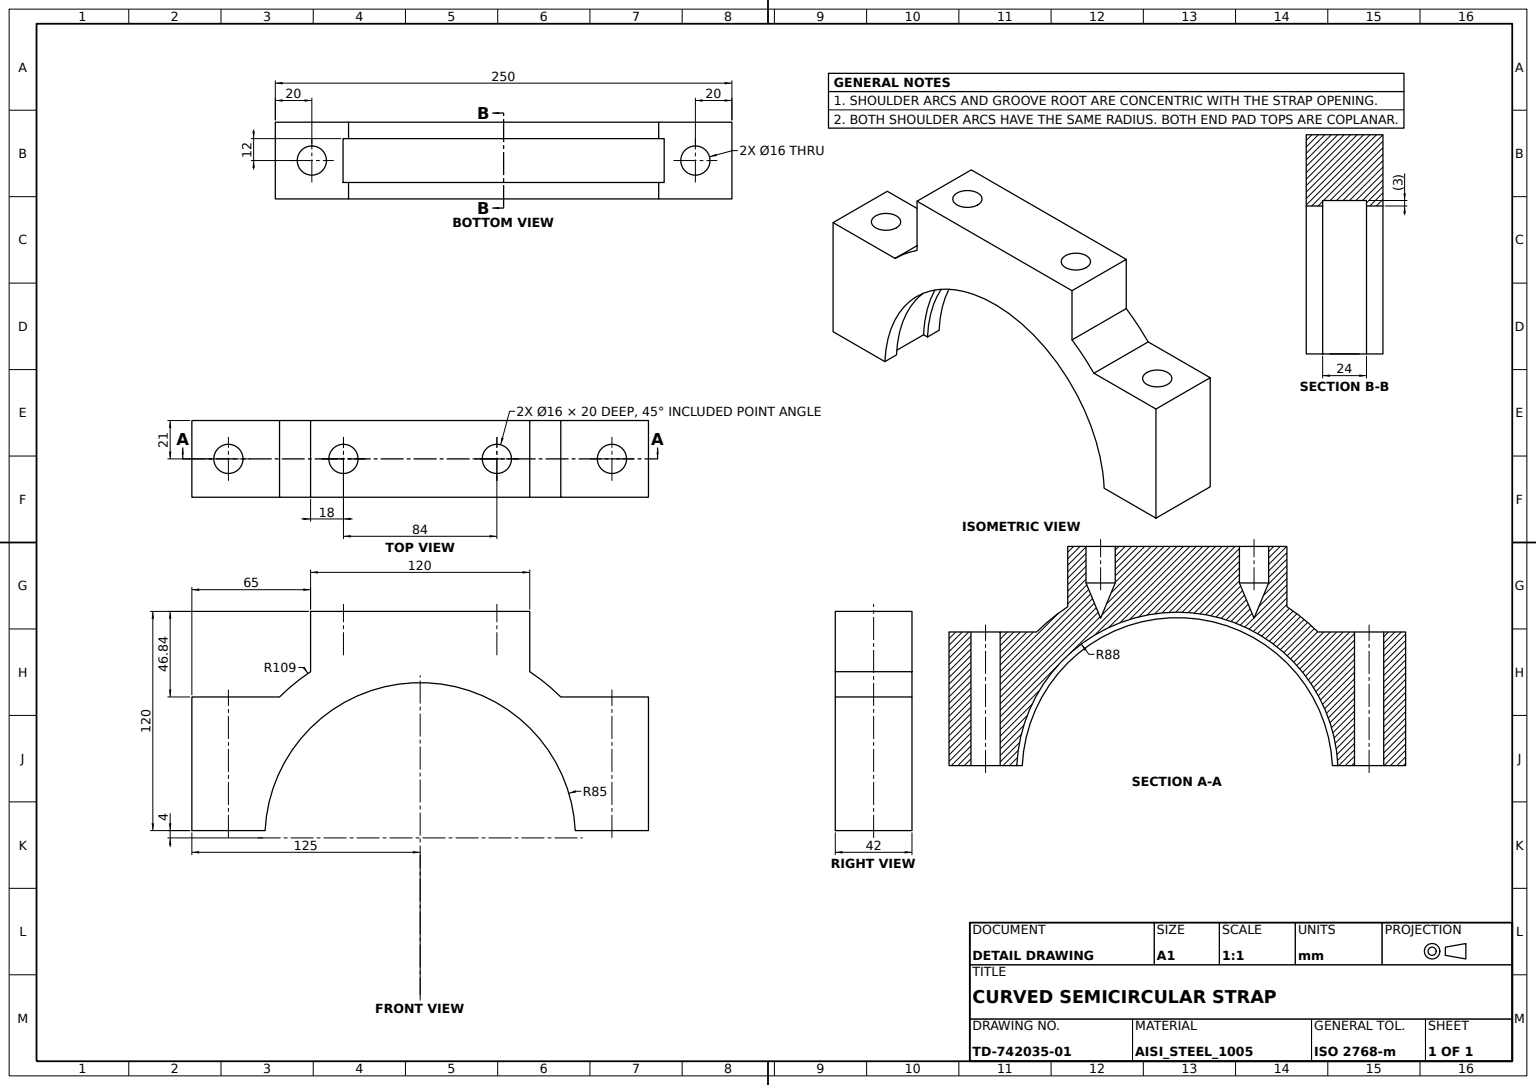
ISO-10303-21;
HEADER;
FILE_DESCRIPTION((''),'2;1');
FILE_NAME('','',(''),(''),'','','');
FILE_SCHEMA(('AUTOMOTIVE_DESIGN'));
ENDSEC;
DATA;
#1=APPLICATION_CONTEXT('');
#2=PRODUCT_CONTEXT('',#1,'mechanical');
#3=PRODUCT('','','',(#2));
#4=PRODUCT_DEFINITION_FORMATION('','',#3);
#5=PRODUCT_DEFINITION_CONTEXT('',#1,'design');
#6=PRODUCT_DEFINITION('','',#4,#5);
#7=PRODUCT_DEFINITION_SHAPE('','',#6);
#8=(LENGTH_UNIT()NAMED_UNIT(*)SI_UNIT(.MILLI.,.METRE.));
#9=(NAMED_UNIT(*)PLANE_ANGLE_UNIT()SI_UNIT($,.RADIAN.));
#10=(NAMED_UNIT(*)SI_UNIT($,.STERADIAN.)SOLID_ANGLE_UNIT());
#11=UNCERTAINTY_MEASURE_WITH_UNIT(LENGTH_MEASURE(0.005),#8,'distance_accuracy_value','');
#12=(GEOMETRIC_REPRESENTATION_CONTEXT(3)GLOBAL_UNCERTAINTY_ASSIGNED_CONTEXT((#11))GLOBAL_UNIT_ASSIGNED_CONTEXT((#8,#9,#10))REPRESENTATION_CONTEXT('',''));
#13=CARTESIAN_POINT('',(0.,-84.90583,-12.));
#14=VERTEX_POINT('',#13);
#15=CARTESIAN_POINT('',(0.,-84.90583,-21.));
#16=VERTEX_POINT('',#15);
#17=CARTESIAN_POINT('',(0.,-84.90583,21.));
#18=DIRECTION('',(0.,0.,-1.));
#19=VECTOR('',#18,1000.);
#20=LINE('',#17,#19);
#21=EDGE_CURVE('',#14,#16,#20,.T.);
#22=ORIENTED_EDGE('',*,*,#21,.T.);
#23=CARTESIAN_POINT('',(0.,84.90583,-21.));
#24=VERTEX_POINT('',#23);
#25=CARTESIAN_POINT('',(4.,0.,-21.));
#26=DIRECTION('',(0.,1.,0.));
#27=AXIS2_PLACEMENT_3D('',#25,#18,#26);
#28=CIRCLE('',#27,85.);
#29=EDGE_CURVE('',#16,#24,#28,.T.);
#30=ORIENTED_EDGE('',*,*,#29,.T.);
#31=CARTESIAN_POINT('',(0.,84.90583,-12.));
#32=VERTEX_POINT('',#31);
#33=CARTESIAN_POINT('',(0.,84.90583,21.));
#34=LINE('',#33,#19);
#35=EDGE_CURVE('',#32,#24,#34,.T.);
#36=ORIENTED_EDGE('',*,*,#35,.F.);
#37=CARTESIAN_POINT('',(4.,0.,-12.));
#38=AXIS2_PLACEMENT_3D('',#37,#18,#26);
#39=CIRCLE('',#38,85.);
#40=EDGE_CURVE('',#14,#32,#39,.T.);
#41=ORIENTED_EDGE('',*,*,#40,.F.);
#42=EDGE_LOOP('',(#22,#30,#36,#41));
#43=FACE_BOUND('',#42,.T.);
#44=CARTESIAN_POINT('',(4.,0.,21.));
#45=DIRECTION('',(-1.,0.,0.));
#46=AXIS2_PLACEMENT_3D('',#44,#18,#45);
#47=CYLINDRICAL_SURFACE('',#46,85.);
#48=ADVANCED_FACE('',(#43),#47,.F.);
#49=CARTESIAN_POINT('',(0.,-84.90583,12.));
#50=VERTEX_POINT('',#49);
#51=CARTESIAN_POINT('',(0.,84.90583,12.));
#52=VERTEX_POINT('',#51);
#53=CARTESIAN_POINT('',(4.,0.,12.));
#54=AXIS2_PLACEMENT_3D('',#53,#18,#26);
#55=CIRCLE('',#54,85.);
#56=EDGE_CURVE('',#50,#52,#55,.T.);
#57=ORIENTED_EDGE('',*,*,#56,.T.);
#58=VERTEX_POINT('',#33);
#59=EDGE_CURVE('',#58,#52,#34,.T.);
#60=ORIENTED_EDGE('',*,*,#59,.F.);
#61=VERTEX_POINT('',#17);
#62=AXIS2_PLACEMENT_3D('',#44,#18,#26);
#63=CIRCLE('',#62,85.);
#64=EDGE_CURVE('',#61,#58,#63,.T.);
#65=ORIENTED_EDGE('',*,*,#64,.F.);
#66=EDGE_CURVE('',#61,#50,#20,.T.);
#67=ORIENTED_EDGE('',*,*,#66,.T.);
#68=EDGE_LOOP('',(#57,#60,#65,#67));
#69=FACE_BOUND('',#68,.T.);
#70=ADVANCED_FACE('',(#69),#47,.F.);
#71=CARTESIAN_POINT('',(0.,-105.,8.));
#72=VERTEX_POINT('',#71);
#73=CARTESIAN_POINT('',(0.,-105.,0.));
#74=DIRECTION('',(0.,0.,1.));
#75=AXIS2_PLACEMENT_3D('',#73,#45,#74);
#76=CIRCLE('',#75,8.);
#77=EDGE_CURVE('',#72,#72,#76,.T.);
#78=ORIENTED_EDGE('',*,*,#77,.F.);
#79=EDGE_LOOP('',(#78));
#80=FACE_BOUND('',#79,.T.);
#81=CARTESIAN_POINT('',(-73.155687,-97.,0.));
#82=VERTEX_POINT('',#81);
#83=CARTESIAN_POINT('',(-73.155687,-105.,0.));
#84=DIRECTION('',(1.,0.,0.));
#85=AXIS2_PLACEMENT_3D('',#83,#84,#26);
#86=CIRCLE('',#85,8.);
#87=EDGE_CURVE('',#82,#82,#86,.T.);
#88=ORIENTED_EDGE('',*,*,#87,.F.);
#89=EDGE_LOOP('',(#88));
#90=FACE_BOUND('',#89,.T.);
#91=CARTESIAN_POINT('',(7.315569,-105.,0.));
#92=DIRECTION('',(0.,-1.,0.));
#93=AXIS2_PLACEMENT_3D('',#91,#45,#92);
#94=CYLINDRICAL_SURFACE('',#93,8.);
#95=ADVANCED_FACE('',(#80,#90),#94,.F.);
#96=ORIENTED_EDGE('',*,*,#64,.T.);
#97=CARTESIAN_POINT('',(0.,125.,21.));
#98=VERTEX_POINT('',#97);
#99=VECTOR('',#26,1000.);
#100=LINE('',#33,#99);
#101=EDGE_CURVE('',#58,#98,#100,.T.);
#102=ORIENTED_EDGE('',*,*,#101,.T.);
#103=CARTESIAN_POINT('',(-73.155687,125.,21.));
#104=VERTEX_POINT('',#103);
#105=VECTOR('',#45,1000.);
#106=LINE('',#97,#105);
#107=EDGE_CURVE('',#98,#104,#106,.T.);
#108=ORIENTED_EDGE('',*,*,#107,.T.);
#109=CARTESIAN_POINT('',(-73.155687,76.993506,21.));
#110=VERTEX_POINT('',#109);
#111=VECTOR('',#92,1000.);
#112=LINE('',#103,#111);
#113=EDGE_CURVE('',#104,#110,#112,.T.);
#114=ORIENTED_EDGE('',*,*,#113,.T.);
#115=CARTESIAN_POINT('',(-87.,60.,21.));
#116=VERTEX_POINT('',#115);
#117=AXIS2_PLACEMENT_3D('',#44,#74,#26);
#118=CIRCLE('',#117,109.);
#119=EDGE_CURVE('',#110,#116,#118,.T.);
#120=ORIENTED_EDGE('',*,*,#119,.T.);
#121=CARTESIAN_POINT('',(-120.,60.,21.));
#122=VERTEX_POINT('',#121);
#123=LINE('',#115,#105);
#124=EDGE_CURVE('',#116,#122,#123,.T.);
#125=ORIENTED_EDGE('',*,*,#124,.T.);
#126=CARTESIAN_POINT('',(-120.,-60.,21.));
#127=VERTEX_POINT('',#126);
#128=LINE('',#121,#111);
#129=EDGE_CURVE('',#122,#127,#128,.T.);
#130=ORIENTED_EDGE('',*,*,#129,.T.);
#131=CARTESIAN_POINT('',(-87.,-60.,21.));
#132=VERTEX_POINT('',#131);
#133=VECTOR('',#84,1000.);
#134=LINE('',#126,#133);
#135=EDGE_CURVE('',#127,#132,#134,.T.);
#136=ORIENTED_EDGE('',*,*,#135,.T.);
#137=CARTESIAN_POINT('',(-73.155687,-76.993506,21.));
#138=VERTEX_POINT('',#137);
#139=EDGE_CURVE('',#132,#138,#118,.T.);
#140=ORIENTED_EDGE('',*,*,#139,.T.);
#141=CARTESIAN_POINT('',(-73.155687,-125.,21.));
#142=VERTEX_POINT('',#141);
#143=LINE('',#137,#111);
#144=EDGE_CURVE('',#138,#142,#143,.T.);
#145=ORIENTED_EDGE('',*,*,#144,.T.);
#146=CARTESIAN_POINT('',(0.,-125.,21.));
#147=VERTEX_POINT('',#146);
#148=LINE('',#141,#133);
#149=EDGE_CURVE('',#142,#147,#148,.T.);
#150=ORIENTED_EDGE('',*,*,#149,.T.);
#151=LINE('',#146,#99);
#152=EDGE_CURVE('',#147,#61,#151,.T.);
#153=ORIENTED_EDGE('',*,*,#152,.T.);
#154=EDGE_LOOP('',(#96,#102,#108,#114,#120,#125,#130,#136,#140,#145,#150,#153));
#155=FACE_BOUND('',#154,.T.);
#156=AXIS2_PLACEMENT_3D('',#44,#74,#84);
#157=PLANE('',#156);
#158=ADVANCED_FACE('',(#155),#157,.T.);
#159=CARTESIAN_POINT('',(-87.,60.,-21.));
#160=VERTEX_POINT('',#159);
#161=LINE('',#115,#19);
#162=EDGE_CURVE('',#116,#160,#161,.T.);
#163=ORIENTED_EDGE('',*,*,#162,.F.);
#164=ORIENTED_EDGE('',*,*,#119,.F.);
#165=CARTESIAN_POINT('',(-73.155687,76.993506,-21.));
#166=VERTEX_POINT('',#165);
#167=LINE('',#109,#19);
#168=EDGE_CURVE('',#110,#166,#167,.T.);
#169=ORIENTED_EDGE('',*,*,#168,.T.);
#170=AXIS2_PLACEMENT_3D('',#25,#74,#26);
#171=CIRCLE('',#170,109.);
#172=EDGE_CURVE('',#166,#160,#171,.T.);
#173=ORIENTED_EDGE('',*,*,#172,.T.);
#174=EDGE_LOOP('',(#163,#164,#169,#173));
#175=FACE_BOUND('',#174,.T.);
#176=CYLINDRICAL_SURFACE('',#46,109.);
#177=ADVANCED_FACE('',(#175),#176,.T.);
#178=CARTESIAN_POINT('',(-120.,60.,-21.));
#179=VERTEX_POINT('',#178);
#180=CARTESIAN_POINT('',(-120.,-60.,-21.));
#181=VERTEX_POINT('',#180);
#182=LINE('',#178,#111);
#183=EDGE_CURVE('',#179,#181,#182,.T.);
#184=ORIENTED_EDGE('',*,*,#183,.T.);
#185=LINE('',#126,#19);
#186=EDGE_CURVE('',#127,#181,#185,.T.);
#187=ORIENTED_EDGE('',*,*,#186,.F.);
#188=ORIENTED_EDGE('',*,*,#129,.F.);
#189=LINE('',#121,#19);
#190=EDGE_CURVE('',#122,#179,#189,.T.);
#191=ORIENTED_EDGE('',*,*,#190,.T.);
#192=EDGE_LOOP('',(#184,#187,#188,#191));
#193=FACE_BOUND('',#192,.T.);
#194=CARTESIAN_POINT('',(-120.,-34.,0.));
#195=VERTEX_POINT('',#194);
#196=CARTESIAN_POINT('',(-120.,-42.,0.));
#197=AXIS2_PLACEMENT_3D('',#196,#84,#26);
#198=CIRCLE('',#197,8.);
#199=EDGE_CURVE('',#195,#195,#198,.T.);
#200=ORIENTED_EDGE('',*,*,#199,.T.);
#201=EDGE_LOOP('',(#200));
#202=FACE_BOUND('',#201,.T.);
#203=CARTESIAN_POINT('',(-120.,50.,0.));
#204=VERTEX_POINT('',#203);
#205=CARTESIAN_POINT('',(-120.,42.,0.));
#206=AXIS2_PLACEMENT_3D('',#205,#84,#26);
#207=CIRCLE('',#206,8.);
#208=EDGE_CURVE('',#204,#204,#207,.T.);
#209=ORIENTED_EDGE('',*,*,#208,.T.);
#210=EDGE_LOOP('',(#209));
#211=FACE_BOUND('',#210,.T.);
#212=AXIS2_PLACEMENT_3D('',#121,#84,#26);
#213=PLANE('',#212);
#214=ADVANCED_FACE('',(#193,#202,#211),#213,.F.);
#215=CARTESIAN_POINT('',(-100.,50.,0.));
#216=VERTEX_POINT('',#215);
#217=CARTESIAN_POINT('',(-100.,42.,0.));
#218=AXIS2_PLACEMENT_3D('',#217,#84,#26);
#219=CIRCLE('',#218,8.);
#220=EDGE_CURVE('',#216,#216,#219,.F.);
#221=ORIENTED_EDGE('',*,*,#220,.T.);
#222=EDGE_LOOP('',(#221));
#223=FACE_BOUND('',#222,.T.);
#224=CARTESIAN_POINT('',(-80.686292,42.,0.));
#225=VERTEX_POINT('',#224);
#226=VERTEX_LOOP('',#225);
#227=FACE_BOUND('',#226,.T.);
#228=AXIS2_PLACEMENT_3D('',#217,#45,#92);
#229=CONICAL_SURFACE('',#228,8.,0.392699082);
#230=ADVANCED_FACE('',(#223,#227),#229,.F.);
#231=CARTESIAN_POINT('',(-100.,-34.,0.));
#232=VERTEX_POINT('',#231);
#233=CARTESIAN_POINT('',(-100.,-42.,0.));
#234=AXIS2_PLACEMENT_3D('',#233,#84,#26);
#235=CIRCLE('',#234,8.);
#236=EDGE_CURVE('',#232,#232,#235,.T.);
#237=ORIENTED_EDGE('',*,*,#236,.T.);
#238=EDGE_LOOP('',(#237));
#239=FACE_BOUND('',#238,.T.);
#240=ORIENTED_EDGE('',*,*,#199,.F.);
#241=EDGE_LOOP('',(#240));
#242=FACE_BOUND('',#241,.T.);
#243=CYLINDRICAL_SURFACE('',#197,8.);
#244=ADVANCED_FACE('',(#239,#242),#243,.F.);
#245=CARTESIAN_POINT('',(0.,-87.909044,12.));
#246=VERTEX_POINT('',#245);
#247=LINE('',#245,#99);
#248=EDGE_CURVE('',#246,#50,#247,.T.);
#249=ORIENTED_EDGE('',*,*,#248,.F.);
#250=CARTESIAN_POINT('',(0.,87.909044,12.));
#251=VERTEX_POINT('',#250);
#252=AXIS2_PLACEMENT_3D('',#53,#74,#26);
#253=CIRCLE('',#252,88.);
#254=EDGE_CURVE('',#246,#251,#253,.F.);
#255=ORIENTED_EDGE('',*,*,#254,.T.);
#256=LINE('',#51,#99);
#257=EDGE_CURVE('',#52,#251,#256,.T.);
#258=ORIENTED_EDGE('',*,*,#257,.F.);
#259=ORIENTED_EDGE('',*,*,#56,.F.);
#260=EDGE_LOOP('',(#249,#255,#258,#259));
#261=FACE_BOUND('',#260,.T.);
#262=AXIS2_PLACEMENT_3D('',#53,#18,#45);
#263=PLANE('',#262);
#264=ADVANCED_FACE('',(#261),#263,.T.);
#265=ORIENTED_EDGE('',*,*,#107,.F.);
#266=CARTESIAN_POINT('',(0.,125.,-21.));
#267=VERTEX_POINT('',#266);
#268=LINE('',#97,#19);
#269=EDGE_CURVE('',#98,#267,#268,.T.);
#270=ORIENTED_EDGE('',*,*,#269,.T.);
#271=CARTESIAN_POINT('',(-73.155687,125.,-21.));
#272=VERTEX_POINT('',#271);
#273=LINE('',#266,#105);
#274=EDGE_CURVE('',#267,#272,#273,.T.);
#275=ORIENTED_EDGE('',*,*,#274,.T.);
#276=LINE('',#103,#19);
#277=EDGE_CURVE('',#104,#272,#276,.T.);
#278=ORIENTED_EDGE('',*,*,#277,.F.);
#279=EDGE_LOOP('',(#265,#270,#275,#278));
#280=FACE_BOUND('',#279,.T.);
#281=AXIS2_PLACEMENT_3D('',#97,#92,#84);
#282=PLANE('',#281);
#283=ADVANCED_FACE('',(#280),#282,.F.);
#284=CARTESIAN_POINT('',(-73.155687,-125.,-21.));
#285=VERTEX_POINT('',#284);
#286=CARTESIAN_POINT('',(0.,-125.,-21.));
#287=VERTEX_POINT('',#286);
#288=LINE('',#284,#133);
#289=EDGE_CURVE('',#285,#287,#288,.T.);
#290=ORIENTED_EDGE('',*,*,#289,.T.);
#291=LINE('',#146,#19);
#292=EDGE_CURVE('',#147,#287,#291,.T.);
#293=ORIENTED_EDGE('',*,*,#292,.F.);
#294=ORIENTED_EDGE('',*,*,#149,.F.);
#295=LINE('',#141,#19);
#296=EDGE_CURVE('',#142,#285,#295,.T.);
#297=ORIENTED_EDGE('',*,*,#296,.T.);
#298=EDGE_LOOP('',(#290,#293,#294,#297));
#299=FACE_BOUND('',#298,.T.);
#300=AXIS2_PLACEMENT_3D('',#141,#26,#45);
#301=PLANE('',#300);
#302=ADVANCED_FACE('',(#299),#301,.F.);
#303=CARTESIAN_POINT('',(0.,105.,8.));
#304=VERTEX_POINT('',#303);
#305=CARTESIAN_POINT('',(0.,105.,0.));
#306=AXIS2_PLACEMENT_3D('',#305,#45,#74);
#307=CIRCLE('',#306,8.);
#308=EDGE_CURVE('',#304,#304,#307,.F.);
#309=ORIENTED_EDGE('',*,*,#308,.T.);
#310=EDGE_LOOP('',(#309));
#311=FACE_BOUND('',#310,.T.);
#312=CARTESIAN_POINT('',(-73.155687,97.,0.));
#313=VERTEX_POINT('',#312);
#314=CARTESIAN_POINT('',(-73.155687,105.,0.));
#315=AXIS2_PLACEMENT_3D('',#314,#45,#92);
#316=CIRCLE('',#315,8.);
#317=EDGE_CURVE('',#313,#313,#316,.T.);
#318=ORIENTED_EDGE('',*,*,#317,.T.);
#319=EDGE_LOOP('',(#318));
#320=FACE_BOUND('',#319,.T.);
#321=CARTESIAN_POINT('',(7.315569,105.,0.));
#322=AXIS2_PLACEMENT_3D('',#321,#45,#92);
#323=CYLINDRICAL_SURFACE('',#322,8.);
#324=ADVANCED_FACE('',(#311,#320),#323,.F.);
#325=ORIENTED_EDGE('',*,*,#186,.T.);
#326=CARTESIAN_POINT('',(-87.,-60.,-21.));
#327=VERTEX_POINT('',#326);
#328=LINE('',#180,#133);
#329=EDGE_CURVE('',#181,#327,#328,.T.);
#330=ORIENTED_EDGE('',*,*,#329,.T.);
#331=LINE('',#131,#19);
#332=EDGE_CURVE('',#132,#327,#331,.T.);
#333=ORIENTED_EDGE('',*,*,#332,.F.);
#334=ORIENTED_EDGE('',*,*,#135,.F.);
#335=EDGE_LOOP('',(#325,#330,#333,#334));
#336=FACE_BOUND('',#335,.T.);
#337=AXIS2_PLACEMENT_3D('',#126,#26,#45);
#338=PLANE('',#337);
#339=ADVANCED_FACE('',(#336),#338,.F.);
#340=ORIENTED_EDGE('',*,*,#236,.F.);
#341=EDGE_LOOP('',(#340));
#342=FACE_BOUND('',#341,.T.);
#343=CARTESIAN_POINT('',(-80.686292,-42.,0.));
#344=VERTEX_POINT('',#343);
#345=VERTEX_LOOP('',#344);
#346=FACE_BOUND('',#345,.T.);
#347=AXIS2_PLACEMENT_3D('',#233,#45,#92);
#348=CONICAL_SURFACE('',#347,8.,0.392699082);
#349=ADVANCED_FACE('',(#342,#346),#348,.F.);
#350=ORIENTED_EDGE('',*,*,#220,.F.);
#351=EDGE_LOOP('',(#350));
#352=FACE_BOUND('',#351,.T.);
#353=ORIENTED_EDGE('',*,*,#208,.F.);
#354=EDGE_LOOP('',(#353));
#355=FACE_BOUND('',#354,.T.);
#356=CYLINDRICAL_SURFACE('',#206,8.);
#357=ADVANCED_FACE('',(#352,#355),#356,.F.);
#358=CARTESIAN_POINT('',(-73.155687,-76.993506,-21.));
#359=VERTEX_POINT('',#358);
#360=EDGE_CURVE('',#327,#359,#171,.T.);
#361=ORIENTED_EDGE('',*,*,#360,.T.);
#362=LINE('',#137,#19);
#363=EDGE_CURVE('',#138,#359,#362,.T.);
#364=ORIENTED_EDGE('',*,*,#363,.F.);
#365=ORIENTED_EDGE('',*,*,#139,.F.);
#366=ORIENTED_EDGE('',*,*,#332,.T.);
#367=EDGE_LOOP('',(#361,#364,#365,#366));
#368=FACE_BOUND('',#367,.T.);
#369=ADVANCED_FACE('',(#368),#176,.T.);
#370=ORIENTED_EDGE('',*,*,#292,.T.);
#371=LINE('',#286,#99);
#372=EDGE_CURVE('',#287,#16,#371,.T.);
#373=ORIENTED_EDGE('',*,*,#372,.T.);
#374=ORIENTED_EDGE('',*,*,#21,.F.);
#375=CARTESIAN_POINT('',(0.,-87.909044,-12.));
#376=VERTEX_POINT('',#375);
#377=LINE('',#375,#99);
#378=EDGE_CURVE('',#376,#14,#377,.T.);
#379=ORIENTED_EDGE('',*,*,#378,.F.);
#380=LINE('',#245,#19);
#381=EDGE_CURVE('',#246,#376,#380,.T.);
#382=ORIENTED_EDGE('',*,*,#381,.F.);
#383=ORIENTED_EDGE('',*,*,#248,.T.);
#384=ORIENTED_EDGE('',*,*,#66,.F.);
#385=ORIENTED_EDGE('',*,*,#152,.F.);
#386=EDGE_LOOP('',(#370,#373,#374,#379,#382,#383,#384,#385));
#387=FACE_BOUND('',#386,.T.);
#388=ORIENTED_EDGE('',*,*,#77,.T.);
#389=EDGE_LOOP('',(#388));
#390=FACE_BOUND('',#389,.T.);
#391=AXIS2_PLACEMENT_3D('',#146,#45,#74);
#392=PLANE('',#391);
#393=ADVANCED_FACE('',(#387,#390),#392,.F.);
#394=ORIENTED_EDGE('',*,*,#378,.T.);
#395=ORIENTED_EDGE('',*,*,#40,.T.);
#396=CARTESIAN_POINT('',(0.,87.909044,-12.));
#397=VERTEX_POINT('',#396);
#398=LINE('',#31,#99);
#399=EDGE_CURVE('',#32,#397,#398,.T.);
#400=ORIENTED_EDGE('',*,*,#399,.T.);
#401=AXIS2_PLACEMENT_3D('',#37,#74,#26);
#402=CIRCLE('',#401,88.);
#403=EDGE_CURVE('',#376,#397,#402,.F.);
#404=ORIENTED_EDGE('',*,*,#403,.F.);
#405=EDGE_LOOP('',(#394,#395,#400,#404));
#406=FACE_BOUND('',#405,.T.);
#407=AXIS2_PLACEMENT_3D('',#37,#18,#45);
#408=PLANE('',#407);
#409=ADVANCED_FACE('',(#406),#408,.F.);
#410=ORIENTED_EDGE('',*,*,#363,.T.);
#411=LINE('',#358,#111);
#412=EDGE_CURVE('',#359,#285,#411,.T.);
#413=ORIENTED_EDGE('',*,*,#412,.T.);
#414=ORIENTED_EDGE('',*,*,#296,.F.);
#415=ORIENTED_EDGE('',*,*,#144,.F.);
#416=EDGE_LOOP('',(#410,#413,#414,#415));
#417=FACE_BOUND('',#416,.T.);
#418=ORIENTED_EDGE('',*,*,#87,.T.);
#419=EDGE_LOOP('',(#418));
#420=FACE_BOUND('',#419,.T.);
#421=AXIS2_PLACEMENT_3D('',#137,#84,#26);
#422=PLANE('',#421);
#423=ADVANCED_FACE('',(#417,#420),#422,.F.);
#424=ORIENTED_EDGE('',*,*,#317,.F.);
#425=EDGE_LOOP('',(#424));
#426=FACE_BOUND('',#425,.T.);
#427=LINE('',#271,#111);
#428=EDGE_CURVE('',#272,#166,#427,.T.);
#429=ORIENTED_EDGE('',*,*,#428,.T.);
#430=ORIENTED_EDGE('',*,*,#168,.F.);
#431=ORIENTED_EDGE('',*,*,#113,.F.);
#432=ORIENTED_EDGE('',*,*,#277,.T.);
#433=EDGE_LOOP('',(#429,#430,#431,#432));
#434=FACE_BOUND('',#433,.T.);
#435=AXIS2_PLACEMENT_3D('',#103,#84,#26);
#436=PLANE('',#435);
#437=ADVANCED_FACE('',(#426,#434),#436,.F.);
#438=ORIENTED_EDGE('',*,*,#329,.F.);
#439=ORIENTED_EDGE('',*,*,#183,.F.);
#440=LINE('',#159,#105);
#441=EDGE_CURVE('',#160,#179,#440,.T.);
#442=ORIENTED_EDGE('',*,*,#441,.F.);
#443=ORIENTED_EDGE('',*,*,#172,.F.);
#444=ORIENTED_EDGE('',*,*,#428,.F.);
#445=ORIENTED_EDGE('',*,*,#274,.F.);
#446=LINE('',#23,#99);
#447=EDGE_CURVE('',#24,#267,#446,.T.);
#448=ORIENTED_EDGE('',*,*,#447,.F.);
#449=ORIENTED_EDGE('',*,*,#29,.F.);
#450=ORIENTED_EDGE('',*,*,#372,.F.);
#451=ORIENTED_EDGE('',*,*,#289,.F.);
#452=ORIENTED_EDGE('',*,*,#412,.F.);
#453=ORIENTED_EDGE('',*,*,#360,.F.);
#454=EDGE_LOOP('',(#438,#439,#442,#443,#444,#445,#448,#449,#450,#451,#452,#453));
#455=FACE_BOUND('',#454,.T.);
#456=AXIS2_PLACEMENT_3D('',#25,#74,#84);
#457=PLANE('',#456);
#458=ADVANCED_FACE('',(#455),#457,.F.);
#459=ORIENTED_EDGE('',*,*,#441,.T.);
#460=ORIENTED_EDGE('',*,*,#190,.F.);
#461=ORIENTED_EDGE('',*,*,#124,.F.);
#462=ORIENTED_EDGE('',*,*,#162,.T.);
#463=EDGE_LOOP('',(#459,#460,#461,#462));
#464=FACE_BOUND('',#463,.T.);
#465=AXIS2_PLACEMENT_3D('',#115,#92,#84);
#466=PLANE('',#465);
#467=ADVANCED_FACE('',(#464),#466,.F.);
#468=ORIENTED_EDGE('',*,*,#254,.F.);
#469=ORIENTED_EDGE('',*,*,#381,.T.);
#470=ORIENTED_EDGE('',*,*,#403,.T.);
#471=LINE('',#250,#19);
#472=EDGE_CURVE('',#251,#397,#471,.T.);
#473=ORIENTED_EDGE('',*,*,#472,.F.);
#474=EDGE_LOOP('',(#468,#469,#470,#473));
#475=FACE_BOUND('',#474,.T.);
#476=CYLINDRICAL_SURFACE('',#262,88.);
#477=ADVANCED_FACE('',(#475),#476,.F.);
#478=ORIENTED_EDGE('',*,*,#308,.F.);
#479=EDGE_LOOP('',(#478));
#480=FACE_BOUND('',#479,.T.);
#481=ORIENTED_EDGE('',*,*,#472,.T.);
#482=ORIENTED_EDGE('',*,*,#399,.F.);
#483=ORIENTED_EDGE('',*,*,#35,.T.);
#484=ORIENTED_EDGE('',*,*,#447,.T.);
#485=ORIENTED_EDGE('',*,*,#269,.F.);
#486=ORIENTED_EDGE('',*,*,#101,.F.);
#487=ORIENTED_EDGE('',*,*,#59,.T.);
#488=ORIENTED_EDGE('',*,*,#257,.T.);
#489=EDGE_LOOP('',(#481,#482,#483,#484,#485,#486,#487,#488));
#490=FACE_BOUND('',#489,.T.);
#491=AXIS2_PLACEMENT_3D('',#33,#45,#74);
#492=PLANE('',#491);
#493=ADVANCED_FACE('',(#480,#490),#492,.F.);
#494=CLOSED_SHELL('',(#48,#70,#95,#158,#177,#214,#230,#244,#264,#283,#302,#324,#339,#349,#357,#369,#393,#409,#423,#437,#458,#467,#477,#493));
#495=MANIFOLD_SOLID_BREP('',#494);
#496=ADVANCED_BREP_SHAPE_REPRESENTATION('',(#495),#12);
#497=SHAPE_DEFINITION_REPRESENTATION(#7,#496);
ENDSEC;
END-ISO-10303-21;
